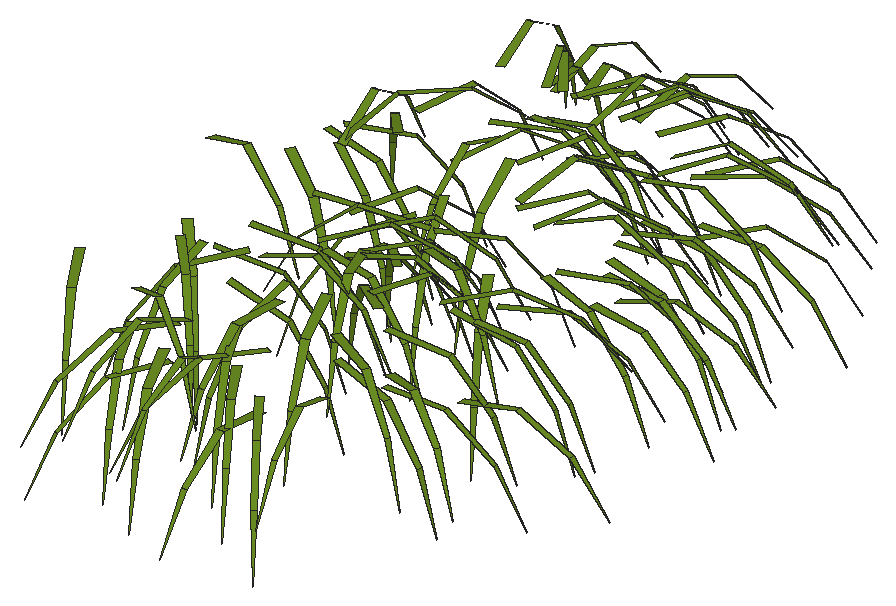
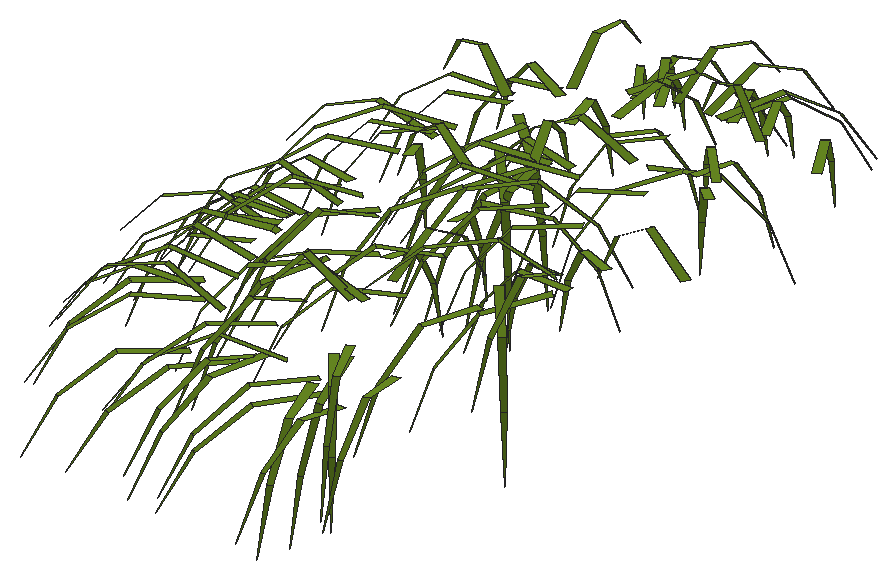
# SketchUp Ruby script. Lengths in inches.
U = 1.inch
M = Sketchup.active_model
def pt(a) = Geom::Point3d.new(a.map { |v| v * U })
def face(e, loops, mat)
  f = e.add_face(loops[0].map { |a| pt(a) })
  loops[1..].each { |l| e.add_face(l.map { |a| pt(a) }).erase! }
  f.material = f.back_material = mat if mat
  f
end
# faces: each face lists its corners as indices into pts; further lists are holes
def faces(e, pts, list, mat = nil) = list.each { |f| face(e, (f[0].is_a?(Array) ? f : [f]).map { |l| l.map { |i| pts[i] } }, mat) }
# xy, xz, yz: faces in a plane at the given z, y or x. An outline is a flat list of corners, or four numbers for a rectangle; further outlines are holes
def ring(l) = l.size == 4 ? [[l[0], l[1]], [l[2], l[1]], [l[2], l[3]], [l[0], l[3]]] : l.each_slice(2).to_a
def flat(e, list, mat, &to3) = list.each { |f| face(e, (f[0].is_a?(Array) ? f : [f]).map { |l| ring(l).map { |u, v| to3.(u, v) } }, mat) }
def xy(e, z, list, mat = nil) = flat(e, list, mat) { |x, y| [x, y, z] }
def xz(e, y, list, mat = nil) = flat(e, list, mat) { |x, z| [x, y, z] }
def yz(e, x, list, mat = nil) = flat(e, list, mat) { |y, z| [x, y, z] }
def lines(e, pts, list) = list.each { |a, b| e.add_line(pt(pts[a]), pt(pts[b])) }
# prism: a flat outline (further loops are holes) pulled along v
def prism(e, loops, v, mat = nil)
  f = face(e, loops, mat); d = Geom::Vector3d.new(v.map { |x| x * U })
  f.pushpull(f.normal.samedirection?(d) ? d.length : -d.length)
end
def box(e, o, s, mat = nil) = prism(e, [[o, [o[0] + s[0], o[1], o[2]], [o[0] + s[0], o[1] + s[1], o[2]], [o[0], o[1] + s[1], o[2]]]], [0, 0, s[2]], mat)
def at(x, y, z, deg = 0) = Geom::Transformation.translation(pt([x, y, z])) * Geom::Transformation.rotation(ORIGIN, Z_AXIS, deg.degrees)
def axes(o, x, y, z) = Geom::Transformation.new([*x, 0, *y, 0, *z, 0, *pt(o).to_a, 1])
def part(name) = M.definitions.add(name)
# library, detail: a bought-in or finely detailed component or shape, given as its bounding box
def library(name, o, s) = part(name).tap { |d| box(d.entities, o, s) }
def detail(e, o, s) = box(e.add_group.entities, o, s)
def put(e, d, t, mat = nil) = e.add_instance(d, t).tap { |i| i.material = mat if mat }
def group(e, t, mat = nil) = e.add_group.tap { |g| g.transformation = t; g.material = mat if mat }.entities
root = M.entities
M.materials.add("[0061_OliveDrab]").color = [107, 142, 35]
p = [[574.92,14.09,556.13],[574.74,13.98,556.13],[575.21,13.41,553.61],[577.11,15.8,556.13],[577.15,15.59,556.13],[577.89,15.86,553.63],
  [578.15,25.27,556.14],[578.18,25.0625,556.14],[579.09,25.28,553.6875],[573.4375,3.7,556.05],[573.29,3.59,556.05],[574.125,2.61,553.76],
  [576.21,9.42,556.24],[576.18,9.22,556.24],[577.07,9.1875,553.77],[570.125,11.77,556.36],[570.16,11.57,556.36],[570.86,11.78,553.83],
  [567.54,14.91,556.36],[567.66,14.73,556.36],[568.21,15.21,553.83],[570.03,16.95,556.36],[569.86,16.88,556.36],[570.23,16.25,553.83],
  [579.75,19.83,555.97],[579.72,19.62,555.97],[581.16,19.51,553.78],[578.88,21.61,556.16],[578.85,21.41,556.16],[579.98,21.35,553.79],
  [565.14,10.8125,556.38],[564.98,10.66,556.38],[565.56,10.2,553.86],[569.63,20.12,556.46],[569.43,20.07,556.46],[569.71,19.36,553.94],
  [577.89,29.84,556.15],[578.05,29.7,556.15],[578.82,30.72,553.86],[564.6,33.53,556.4],[564.79,33.58,556.4],[564.47,34.41,553.93],
  [575.05,34.09,556.14],[575.22,33.95,556.14],[575.95,35.05,553.87],[567.74,8.3,556.53],[567.54,8.32,556.53],[567.58,7.54,554.03],
  [566.66,19.29,556.52],[566.57,19.125,556.52],[567.29,18.84,554.01],[579.34,27.34,556.16],[579.35,27.13,556.16],[580.82,27.31,553.99],
  [568.4375,3.41,556.46],[568.23,3.31,556.46],[568.79,2.41,554.05],[565.57,15.91,556.61],[565.42,16.08,556.61],[564.93,15.45,554.11],
  [579.36,21.49,556.38],[579.35,21.27,556.38],[580.7,21.3125,554.12],[578.45,24.08,556.47],[578.49,23.88,556.47],[579.55,24.24,554.1],
  [577.89,15.69,556.66],[577.92,15.49,556.66],[578.87,15.71,554.22],[570.02,18.79,556.71],[570.21,18.7,556.71],[570.45,19.48,554.21],
  [564.32,8.57,556.8],[564.12,8.55,556.8],[564.28,7.73,554.3125],[567.35,18.5,556.79],[567.5,18.64,556.79],[566.86,19.18,554.3],
  [572.24,21.56,556.8],[572.4,21.43,556.8],[572.86,22.14,554.31],[565.34,25.29,556.77],[565.5,25.125,556.77],[566.01,25.78,554.28],
  [561.49,26.04,556.75],[561.64,26.18,556.75],[561.01,26.74,554.27],[568.48,34.6875,556.49],[568.65,34.57,556.49],[569.36,35.76,554.26],
  [578.55,10.67,556.64],[578.56,10.49,556.64],[579.93,10.64,554.41],[568.14,15.58,556.86],[568.28,15.75,556.86],[567.54,16.22,554.38],
  [565.65,17.61,556.85],[565.53,17.42,556.85],[566.32,17.05,554.37],[565.4,2.66,556.76],[565.22,2.73,556.76],[564.88,1.48,554.48],
  [562.55,10.13,556.99],[562.4,10.29,556.99],[561.84,9.58,554.52],[576.72,12.9,556.96],[576.75,12.68,556.96],[577.67,12.91,554.51],
  [568.54,19.62,556.99],[568.62,19.44,556.99],[569.39,19.89,554.52],[577.96,22.03,556.79],[578.05,21.86,556.79],[579.125,22.52,554.49],
  [573.97,27.52,557],[574.07,27.34,557],[574.8,27.84,554.53],[564.69,35.09,556.68],[564.9,35.16,556.68],[564.31,36.45,554.47],
  [566.89,3.82,556.9375],[566.71,3.72,556.9375],[567.375,2.71,554.6],[571.23,8.54,557.1],[571.03,8.46,557.1],[571.47,7.66,554.63],
  [580.23,12.86,556.61],[580.23,12.65,556.61],[581.93,12.74,554.62],[568.47,15.9,557.05],[568.52,15.7,557.05],[569.36,16.02,554.58],
  [571.49,2.26,556.85],[571.26,2.24,556.85],[571.53,0.71,554.74],[578.4,18.14,556.89],[578.35,17.94,556.89],[579.7,17.68,554.65],
  [568.37,18.78,557.16],[568.59,18.79,557.16],[568.42,19.71,554.7],[571.95,29.11,557.16],[572.13,29.03,557.16],[572.4375,29.9,554.7],
  [572.17,34.87,556.87],[572.36,34.76,556.87],[573.0625,36.13,554.75],[571.97,3.97,557.11],[571.8,3.85,557.11],[572.61,2.83,554.83],
  [566.53,21.2,557.25],[566.51,21,557.25],[567.46,20.97,554.81],[576.82,31.375,557.02],[576.93,31.21,557.02],[578.07,32.14,554.84],
  [568.62,34.58,557.08],[568.78,34.48,557.08],[569.36,35.65,554.8],[570.48,19.67,557.37],[570.65,19.59,557.37],[570.99,20.49,554.93],
  [569.56,35.09,557.07],[569.76,35.05,557.07],[569.95,36.55,554.92],[563.1875,6.04,557.43],[563.01,5.93,557.43],[563.64,5.13,555.01],
  [575.34,8.76,557.42],[575.24,8.57,557.42],[576.24,8.16,555.03],[563.45,33.1875,557.41],[563.61,33.3125,557.41],[562.83,34.17,555.05],
  [570.5,5.33,557.44],[570.33,5.23,557.44],[571.02,4.22,555.12],[571.82,17.82,557.54],[572.02,17.76,557.54],[572.2,18.76,555.12],
  [578.21,18.48,557.33],[578.29,18.29,557.33],[579.48,18.88,555.0625],[580.15,22.01,557.05],[580.16,21.8125,557.05],[581.91,22.02,555.1],
  [578.45,25.16,557.44],[578.52,24.95,557.44],[579.85,25.51,555.24],[570.375,27.55,557.64],[570.45,27.38,557.64],[571.37,27.91,555.23],
  [566.15,9.24,557.67],[566.01,9.11,557.67],[566.87,8.33,555.3125],[563.74,33.125,557.7],[563.9,33.21,557.7],[563.28,34.16,555.33],
  [571.99,13.95,557.77],[571.94,13.74,557.77],[573.03,13.6,555.38],[567.82,4.56,557.75],[567.63,4.65,557.75],[567.12,3.44,555.48],
  [564.73,29.06,557.93],[564.94,29.01,557.93],[565.07,30.09,555.53],[564.46,35.79,557.53],[564.65,35.81,557.53],[564.4,37.52,555.55],
  [568.87,6.47,558.06],[568.65,6.46,558.06],[568.8125,5.27,555.73],[573.43,25.23,558.03],[573.6,25.11,558.03],[574.16,26.12,555.67],
  [564.47,3.84,557.96],[564.28,3.92,557.96],[563.82,2.58,555.75],[577.35,26.47,558.14],[577.35,26.26,558.14],[578.68,26.4,555.88],
  [572.28,5.35,557.73],[572.07,5.19,557.73],[577.87,8.35,558.08],[577.76,8.16,558.08],[579.22,7.39,556.04],[570.75,11.59,558.36],
  [570.55,11.5,558.36],[571.17,10.47,556.03],[572.71,16.73,558.27],[572.79,16.52,558.27],[573.94,17.05,555.97],[577.63,20.2,557.47],
  [577.58,19.89,557.47],[568.6875,21.68,558.32],[568.86,21.58,558.32],[569.35,22.71,556],[562.27,34.2,558.15],[562.45,34.25,558.15],
  [561.99,35.64,555.98],[574.21,15.35,558.32],[573.95,15.19,558.32],[575.625,15.53,558.28],[575.6875,15.24,558.28],[576.45,25.1,558.13],
  [576.49,24.81,558.13],[571.89,26.17,558.38],[571.86,25.97,558.38],[573.08,25.9,556.05],[573.69,32.44,557.67],[573.93,32.25,557.67],
  [574.58,9.72,558.28],[574.54,9.42,558.28],[574.53,15.11,558.47],[574.43,14.92,558.47],[575.625,14.43,556.18],[577.02,21.92,557.98],
  [576.97,21.64,557.98],[577.16,27.27,557.62],[577.18,26.98,557.62],[576.45,28.3,557.72],[576.68,28.1,557.72],[569.46,35.34,558.16],
  [569.66,35.32,558.16],[569.75,37.03,556.17],[565.28,16.19,558.59],[565.2,16.36,558.59],[564.14,15.74,556.27],[571.73,33.21,558.41],
  [571.84,33.06,558.41],[573.08,34.07,556.33],[571.71,33.48,558.32],[571.87,33.38,558.32],[572.64,34.8125,556.26],[574.18,3.92,558.24],
  [573.99,3.86,558.24],[574.65,2.14,556.37],[564.2,11.91,558.57],[563.97,11.7,558.57],[568.7,11.61,558.55],[568.74,11.32,558.55],
  [566.32,14.17,558.56],[566.49,13.91,558.56],[569.49,18.29,558.55],[569.25,18.18,558.55],[571.67,19.27,558.7],[571.77,19.08,558.7],
  [572.79,19.79,556.39],[577.28,21.64,557.96],[577.26,21.33,557.96],[571.39,27.9,558.64],[571.55,27.79,558.64],[572.17,28.95,556.36],
  [564.97,31.92,558.44],[565.25,31.99,558.44],[567.66,5.11,558.3],[567.375,4.97,558.3],[567.89,9.8,558.68],[567.61,9.82,558.68],
  [565.37,20.04,558.68],[565.24,19.81,558.68],[569.32,21.56,558.63],[569.03,21.49,558.63],[576.59,23.67,558.29],[576.66,23.39,558.29],
  [567.22,32.98,558.03],[567.46,32.81,558.03],[576.43,10.62,558.19],[576.44,10.36,558.19],[577.83,12.93,557.68],[577.83,12.63,557.68],
  [566.71,16.94,558.74],[566.49,17.17,558.74],[576.63,29.7,558.71],[576.74,29.52,558.71],[578.02,30.38,556.59],[576.125,15.52,558.59],
  [576.16,15.23,558.59],[563.84,17.13,559.01],[563.77,16.93,559.01],[565.03,16.57,556.73],[569.34,17.38,558.8125],[569.6,17.26,558.8125],
  [570.74,18.15,558.91],[570.86,17.97,558.91],[571.96,18.89,556.7],[577.08,22.28,558.94],[577.11,22.08,558.94],[578.43,22.33,556.69],
  [565.39,33.06,558.2],[565.68,33.16,558.2],[569.06,3.03,558.8],[568.87,3.01,558.8],[569.13,1.33,556.8],[566.12,4.625,558.35],
  [565.87,4.71,558.35],[564.24,10.17,558.88],[563.96,10.15,558.88],[568.41,17.3,558.875],[568.61,17.49,558.875],[564.31,18.52,558.91],
  [564.14,18.26,558.91],[568.03,20.36,559.04],[567.84,20.34,559.04],[568.09,19.01,556.79],[571.18,20.37,558.88],[571.4,20.18,558.88],
  [576.15,21.16,558.48],[576.27,20.91,558.48],[564.18,24.2,558.86],[564.4,23.98,558.86],[575.35,24.24,559],[575.49,24.1,559],
  [576.375,25.14,556.75],[562.51,24.8125,558.83],[562.73,25,558.83],[566.22,3.74,559.01],[566,3.76,559.01],[565.96,2.25,556.86],
  [571.31,4.5625,558.11],[570.99,4.53,558.11],[565.97,5.59,558.64],[565.71,5.45,558.64],[570.82,13.06,559.1],[570.81,12.84,559.1],
  [572.1875,12.87,556.86],[569.38,14.49,558.9],[569.59,14.73,558.9],[576.4,18.73,558.49],[576.33,18.44,558.49],[562.47,25.65,559.15],
  [562.65,25.68,559.15],[562.35,26.94,556.87],[572.42,26.09,559.02],[572.38,25.88,559.02],[573.86,25.7,556.86],[569.6,26.64,559.09],
  [569.76,26.53,559.09],[570.47,27.82,556.92],[576.55,29.61,558.89],[576.57,29.43,558.89],[578.27,29.72,556.91],[569.8,32.5,559.12],
  [569.98,32.47,559.12],[570.13,33.89,556.92],[570.97,32.96,558.2],[571.23,32.8,558.2],[567.95,6.51,559.07],[567.85,6.34,559.07],
  [569.21,5.59,556.96],[563.77,11.28,559.01],[563.55,11.5,559.01],[574.97,12.73,558.91],[575.01,12.41,558.91],[576.4,12.63,557.35],
  [576.91,17.52,558.92],[577.03,17.33,558.92],[578.45,18.33,556.95],[566.99,18.98,559.01],[567.1,18.73,559.01],[577.7,21.89,557.99],
  [577.72,21.62,557.99],[571.93,26.28,559.21],[572.15,26.21,559.21],[572.4375,27.55,556.97],[572.46,26.8,559.02],[572.6,26.53,559.02],
  [575,30.14,558.45],[575.16,29.91,558.45],[570.85,5.73,558.7],[570.6,5.57,558.7],[570.65,10.14,559.09],[570.36,10.03,559.09],
  [575.28,12.99,557.1],[575.27,12.625,557.1],[566.83,15.52,559.07],[566.9,15.23,559.07],[567.51,32.77,558.63],[567.74,32.64,558.63],
  [569.09,32.93,558.49],[569.38,32.88,558.49],[568.43,17.06,559.14],[568.73,17.08,559.14],[575.2,21.77,557.1875],[575.22,21.43,557.1875],
  [571.17,27.58,559.14],[571.42,27.46,559.14],[576.23,17.72,558.875],[576.34,17.46,558.875],[564.8,21.48,559.21],[564.76,21.2,559.21],
  [569.55,7.08,559.15],[569.3125,6.95,559.15],[562.24,7.625,559.3],[561.99,7.47,559.3],[573.68,9.7,559.22],[573.54,9.43,559.22],
  [569.67,18.08,559.29],[569.91,17.96,559.29],[576.35,24.5,558.875],[576.45,24.21,558.875],[572.05,30.42,557.36],[572.34,30.18,557.36],
  [564.64,31.58,559.1],[564.87,31.75,559.1],[571.27,16.06,559.41],[571.55,15.98,559.41],[575.04,20.62,557.49],[574.98,20.24,557.49],
  [574.6875,26.375,557.48],[574.96,26.125,557.48],[564.64,33.38,558.55],[564.91,33.41,558.55],[571.09,7.14,557.64],[570.7,7.1,557.64],
  [568.65,26.79,559.46],[568.76,26.55,559.46],[574.54,27.18,557.65],[574.56,26.81,557.65],[570.76,7.47,558.03],[570.5,7.28,558.03],
  [564.85,10.7,559.42],[564.65,10.51,559.42],[564.66,31.36,559.41],[564.89,31.48,559.41],[568.85,6.43,559.28],[568.58,6.5625,559.28],
  [570.12,14.44,559.54],[570.05,14.15,559.54],[564.28,27.17,559.6875],[564.57,27.1,559.6875],[564.84,30.85,557.89],[565.17,30.88,557.89],
  [565.375,5.85,559.38],[565.09,5.97,559.38],[574.66,21.81,558.03],[574.64,21.43,558.03],[574.44,22.32,558.32],[574.39,21.97,558.32],
  [572.27,23.6,559.72],[572.51,23.43,559.72],[569.59,30.74,557.96],[569.92,30.54,557.96],[565.69,30.85,558.07],[565.98,30.64,558.07],
  [572.72,8.65,558.14],[572.39,8.54,558.14],[573.18,6.21,559.0625],[573.45,6.3,559.0625],[568.83,8.52,559.71],[568.51,8.5,559.71],
  [575.87,9.65,559.17],[575.7,9.38,559.17],[573.89,24.8,558.62],[573.93,24.45,558.62],[575.16,26.46,559.6],[575.17,26.16,559.6],
  [567.01,7.09,558.22],[566.7,7.2,558.22],[573.81,10.53,558.23],[573.82,10.21,558.23],[566.26,30.58,558.22],[566.62,30.71,558.22],
  [562.82,32,559.49],[563.07,32.07,559.49],[569.15,32.93,559.15],[569.42,32.9,559.15],[566.55,7.49,558.43],[566.2,7.32,558.43],
  [572.06,10.14,558.86],[572,9.78,558.86],[573.19,15.04,559.12],[573.26,14.68,559.12],[572.97,17.47,559.25],[572.65,17.27,559.25],
  [570.71,16.08,559.84],[570.8125,15.78,559.84],[567.67,19.85,559.9],[567.91,19.72,559.9],[574.05,23.08,558.54],[574.13,22.74,558.54],
  [572.84,28.65,558.3125],[573.04,28.36,558.3125],[568.83,30.46,558.33],[569.17,30.42,558.33],[570.45,31.5,559.49],[570.67,31.36,559.49],
  [569.88,13.48,559.97],[569.61,13.35,559.97],[569.82,26.5,559.96],[569.78,26.21,559.96],[565.59,29.44,559.03],[565.93,29.53,559.03],
  [568.5625,30.37,558.42],[568.92,30.3,558.42],[566.16,30.54,558.38],[566.4375,30.37,558.38],[569.77,31.83,559.47],[569.92,31.62,559.47],
  [573.73,11.01,558.46],[573.53,10.68,558.46],[572.65,16.13,559.98],[572.51,15.86,559.98],[573.89,19.44,558.71],[573.79,19.1,558.71],
  [573.8,20,558.68],[573.95,19.7,558.68],[571.76,29.13,558.51],[571.8,28.81,558.51],[574.11,29.1,559.73],[574.08,29.37,559.73],
  [567.78,30.42,558.49],[567.97,30.17,558.49],[564.74,7.91,558.71],[564.43,7.74,558.71],[569.42,7.93,558.57],[569.11,7.73,558.57],
  [566.27,11.29,559.5],[566.33,10.93,559.5],[562.57,13.75,559.5],[562.29,13.49,559.5],[564.25,12.86,559.5],[564.45,12.54,559.5],
  [573.53,15.24,558.9],[573.58,14.89,558.9],[567.21,17.1,560.13],[567.09,17.34,560.13],[568.54,20.54,559.5],[568.24,20.41,559.5],
  [568.75,23.97,559.5],[568.39,23.88,559.5],[570.18,26.09,560.11],[570.42,25.9375,560.11],[568.66,7.875,558.67],[568.33,7.84,558.67],
  [568.59,5.45,559.73],[568.86,5.48,559.73],[568.1,12.29,559.5],[567.76,12.3125,559.5],[573.79,16.77,558.7],[573.92,16.45,558.7],
  [568.55,18.65,559.5],[568.28,18.9375,559.5],[569.79,18.23,560.22],[569.9375,17.98,560.22],[563.19,21.26,559.5],[563.1875,21.25,559.5],
  [563.04,20.98,559.5],[573.86,23.7,558.65],[573.98,23.34,558.65],[574.55,28.55,559.82],[574.7,28.3,559.82],[568.26,15.09,559.5],
  [568.3,15.07,559.5],[568.59,14.9375,559.5],[564.16,22.89,559.5],[564.43,23.12,559.5],[572.43,27.37,558.83],[572.61,27.05,558.83],
  [564.08,12.71,559.5],[563.73,12.69,559.5],[572.38,12.43,559.22],[572.43,12.05,559.22],[571.35,12.8125,559.39],[571.59,13.11,559.39],
  [570.12,15.41,559.5],[570.37,15.64,559.5],[574.82,16.29,559.9375],[574.99,16.03,559.9375],[568.87,16.86,560.22],[569.05,16.61,560.22],
  [569.52,18.4375,559.5],[569.79,18.21,559.5],[562.17,19.93,559.5],[561.97,19.61,559.5],[574.84,22.07,560.29],[574.875,21.79,560.29],
  [562.34,22.45,559.5],[562.61,22.17,559.5],[566.49,6.08,560.17],[566.17,6.11,560.17],[566.42,8.24,559.03],[566.08,8.38,559.03],
  [570.08,8.72,559.01],[569.76,8.89,559.01],[569.03,7.44,559.18],[565.625,13.07,559.5],[565.35,13.35,559.5],[561.78,17.95,560.41],
  [561.67,17.67,560.41],[564.61,17.97,559.5],[564.75,17.67,559.5],[567.81,22.6,560.39],[567.54,22.57,560.39],[573.73,22.66,560.33],
  [573.93,22.47,560.33],[570.15,25.64,559.49],[570.32,25.32,559.49],[570.16,26.57,560.27],[570.1,26.28,560.27],[569.07,29.32,558.98],
  [569.35,29.15,558.98],[563.45,29.5,558.99],[563.76,29.59,558.99],[566.21,29.48,558.96],[566.49,29.69,558.96],[565.97,7.81,560.21],
  [565.83,7.58,560.21],[569.72,12.5625,559.5],[569.37,12.42,559.5],[568.56,13.24,560.42],[568.54,12.93,560.42],[564.32,14.89,559.5],
  [564.41,14.55,559.5],[568.54,14.46,559.5],[568.92,14.48,559.5],[568.33,24.71,560.34],[568.56,24.5625,560.34],[570.02,25.25,559.5],
  [570.33,25.1,559.5],[572.6,26.43,559.06],[572.61,26.06,559.06],[569.38,30.23,560.36],[569.64,30.18,560.36],[566.75,8.5,559.17],
  [566.37,8.53,559.17],[568.28,9.375,559.28],[567.99,9.21,559.28],[571.375,10.96,559.24],[571.2,10.64,559.24],[562.22,21.875,559.5],
  [562.18,21.54,559.5],[562.8,23.4375,560.53],[563.0625,23.48,560.53],[571.22,24.12,560.52],[571.52,24.03,560.52],[565.88,29.05,559.21],
  [566.16,29.2,559.21],[560.86,9.86,559.43],[560.56,9.66,559.43],[563.92,9.15,559.28],[563.74,8.87,559.28],[572.64,14.99,559.26],
  [572.84,14.67,559.26],[568.5,15.74,559.5],[568.56,15.71,559.5],[568.8,15.6,559.5],[572.42,21.82,559.32],[572.46,21.48,559.32],
  [568.95,27.85,559.33],[569.27,27.8,559.33],[563.09,12.64,559.5],[562.85,12.42,559.5],[570.52,13.55,559.5],[570.86,13.45,559.5],
  [571.99,20.94,559.39],[572.23,20.7,559.39],[568.75,11.13,559.5],[568.37,11.12,559.5],[566.11,13.42,559.5],[566.08,13.04,559.5],
  [568.79,15.82,559.5],[568.45,15.66,559.5],[567.57,15.08,559.5],[567.49,14.72,559.5],[568.24,15.26,559.5],[568.37,14.89,559.5],
  [566.8,15.41,559.5],[567.02,15.11,559.5],[570.37,17.35,559.5],[570.2,17.01,559.5],[567.58,17,559.5],[567.77,16.6875,559.5],
  [569.51,18.19,559.5],[569.36,18.49,559.5],[566.42,17.58,559.5],[566.72,17.42,559.5],[559.49,18.85,559.5],[559.36,18.5,559.5],
  [563.17,21.06,559.5],[563.49,21.11,559.5],[562.97,21.4375,559.5],[563.26,21.18,559.5],[564.57,22.71,561.18],[564.34,22.92,561.18],
  [570.76,21.46,559.5],[571.07,21.25,559.5],[570.48,21.82,559.5],[570.85,21.7,559.5],[566.97,22.62,559.5],[567.25,22.45,559.5],
  [567.56,25.06,559.5],[567.23,25.02,559.5],[568.78,23.95,559.5],[569.07,23.77,559.5],[563.69,24.61,559.5],[564.05,24.54,559.5],
  [566.26,25.71,559.5],[566.39,25.41,559.5],[567.26,26.89,559.5],[567.21,26.53,559.5],[567.7,27.09,559.5],[567.63,26.73,559.5],
  [566.11,24.85,561.12],[566.28,24.7,561.12],[567.64,26.4,559.64]]
faces(root,p,[[0,1,2],[3,4,5],[6,7,8],[9,10,11],[12,13,14],[15,16,17],[18,19,20],[21,22,23],
  [24,25,26],[27,28,29],[30,31,32],[33,34,35],[36,37,38],[39,40,41],[42,43,44],[45,46,47],
  [48,49,50],[51,52,53],[54,55,56],[57,58,59],[60,61,62],[63,64,65],[66,67,68],[69,70,71],
  [72,73,74],[75,76,77],[78,79,80],[81,82,83],[84,85,86],[87,88,89],[90,91,92],[93,94,95],
  [96,97,98],[99,100,101],[102,103,104],[105,106,107],[108,109,110],[111,112,113],[114,115,116],[117,118,119],
  [120,121,122],[123,124,125],[126,127,128],[129,130,131],[132,133,134],[135,136,137],[138,139,140],[141,142,143],
  [144,145,146],[147,148,149],[150,151,152],[153,154,155],[156,157,158],[159,160,161],[162,163,164],[165,166,167],
  [168,169,170],[171,172,173],[174,175,176],[177,178,179],[180,181,182],[183,184,185],[186,187,188],[189,190,191],
  [192,193,194],[195,196,197],[198,199,200],[201,202,203],[204,205,206],[207,208,209],[210,211,212],[213,214,215],
  [216,217,218],[219,220,221],[222,223,10,9],[224,225,226],[227,228,229],[230,231,232],[233,234,25,24],[235,236,237],
  [238,239,240],[241,242,1,0],[243,244,4,3],[245,246,7,6],[247,248,249],[250,251,43,42],[252,253,13,12],[254,255,256],
  [257,258,28,27],[259,260,52,51],[261,262,37,36],[263,264,265],[266,267,268],[269,270,271],[272,273,274],[275,276,277],
  [278,279,31,30],[280,281,16,15],[282,283,19,18],[284,285,22,21],[286,287,288],[289,290,61,60],[291,292,293],[294,295,40,39],
  [296,297,55,54],[298,299,46,45],[300,301,49,48],[302,303,34,33],[304,305,64,63],[306,307,88,87],[308,309,91,90],[310,311,127,126],
  [312,313,58,57],[314,315,316],[317,318,67,66],[319,320,321],[322,323,70,69],[324,325,326],[327,328,329],[330,331,118,117],
  [332,333,334],[335,336,100,99],[337,338,73,72],[339,340,76,75],[341,342,97,96],[343,344,345],[346,347,79,78],[348,349,112,111],
  [350,351,82,81],[352,353,354],[355,356,85,84],[357,358,359],[360,361,133,132],[362,363,121,120],[364,365,366],[367,368,94,93],
  [369,370,136,135],[371,372,373],[374,375,376],[377,378,379],[380,381,382],[383,384,385],[386,387,145,144],[388,389,390],
  [391,392,103,102],[393,394,395,106,105],[396,397,398],[399,400,109,108],[401,402,184,183],[403,404,405],[406,407,115,114],[408,409,154,153],
  [410,411,148,147],[412,413,124,123],[414,415,395,311,310],[416,417,130,129],[418,419,157,156],[420,421,163,162],[422,423,139,138],[424,425,402,401],
  [426,427,142,141],[428,429,181,180],[430,431,151,150],[432,433,175,174],[434,435,166,165],[436,437,169,168],[438,439,160,159],[440,441,187,186],
  [442,443,251,250],[444,445,172,171],[446,447,178,177],[448,449,234,233],[450,451,262,261],[452,453,208,207],[454,455,361,360],[456,457,190,189],
  [458,459,260,259],[460,461,223,222],[462,463,193,192],[464,465,196,195],[466,467,202,201],[468,469,199,198],[470,471,205,204],[472,473,453,452],
  [474,475,217,216],[476,477,290,289],[478,479,258,257],[480,481,214,213],[482,483,387,386],[484,485,307,306],[486,487,488,489],[490,491,211,210],
  [492,493,225,224],[494,495,246,245],[496,497,220,219],[489,488,276,275],[498,499,336,335],[500,501,309,308],[502,503,331,330],[504,505,239,238],
  [506,507,264,263],[508,509,297,296],[510,511,253,252],[512,513,244,243],[514,515,242,241],[516,517,231,230],[518,519,236,235],[520,521,305,304],
  [522,523,409,408],[524,525,507,506],[526,527,273,272],[528,529,228,227],[530,531,248,247],[532,533,295,294],[534,535,421,420],[536,537,419,418],
  [538,539,270,269],[540,541,493,492],[542,543,255,254],[544,545,370,369],[546,547,349,348],[548,549,550,551],[552,553,539,538],[554,555,363,362],
  [556,557,411,410],[558,559,281,280],[560,561,279,278],[562,563,283,282],[564,565,318,317],[566,567,267,266],[568,569,285,284],[570,571,303,302],
  [572,573,292,291],[574,575,576,577],[578,579,299,298],[580,581,429,428],[582,583,313,312],[584,585,287,286],[586,587,588,301,300],[589,590,441,440],
  [591,592,315,314],[577,576,333,332],[593,594,595,323,322],[596,597,356,355],[598,599,592,591],[600,601,338,337],[602,603,394,393],[604,605,368,367],
  [606,607,340,339],[608,609,397,396],[610,611,325,324],[612,613,347,346],[614,615,342,341],[616,617,328,327],[618,619,351,350],[551,550,381,380],
  [620,621,358,357],[622,623,475,474],[624,625,626,467,466],[627,628,392,391],[629,630,320,319],[631,632,400,399],[633,634,344,343],[635,636,353,352],
  [637,638,407,406],[639,640,375,374],[641,642,527,526],[643,644,505,504],[645,646,445,444],[647,648,389,388],[649,650,413,412],[651,652,365,364],
  [653,654,417,416],[655,656,423,422],[657,658,378,377],[659,660,427,426],[661,662,497,496],[663,664,384,383],[665,666,621,620],[667,668,626,433,432],
  [669,670,437,436],[671,672,431,430],[673,674,372,371],[675,676,404,403],[677,678,465,464],[679,680,435,434],[681,682,648,647],[683,684,609,608],
  [685,686,687,439,438],[688,689,617,616],[690,691,664,663],[692,693,463,462],[694,695,447,446],[696,697,636,635],[698,699,491,490],[700,701,652,651],
  [702,686,703,529,528],[704,705,469,468],[706,594,707,517,516],[708,709,611,610],[710,711,543,542],[712,713,585,584],[714,715,567,566],[716,717,519,518],
  [718,719,630,629],[720,721,674,673],[722,587,723,724,725],[726,727,481,480],[728,729,676,675],[730,731,658,657],[732,733,634,633],[734,735,573,572],
  [736,737,471,470],[738,739,457,456],[740,741,531,530],[742,743,640,639],[744,745,746],[725,724,745,744]],"[0061_OliveDrab]")
